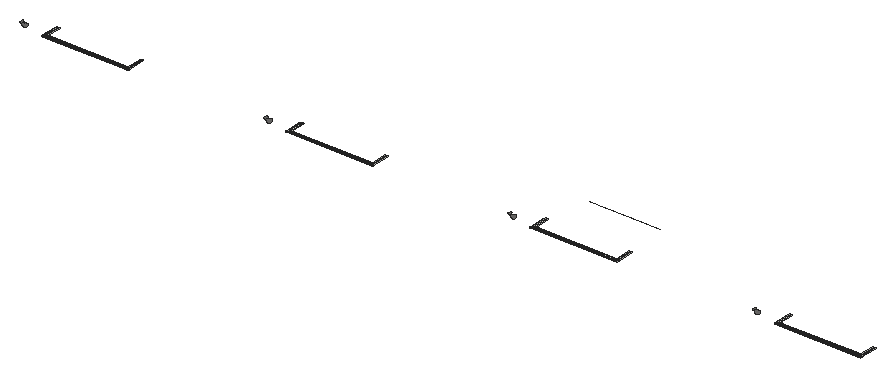
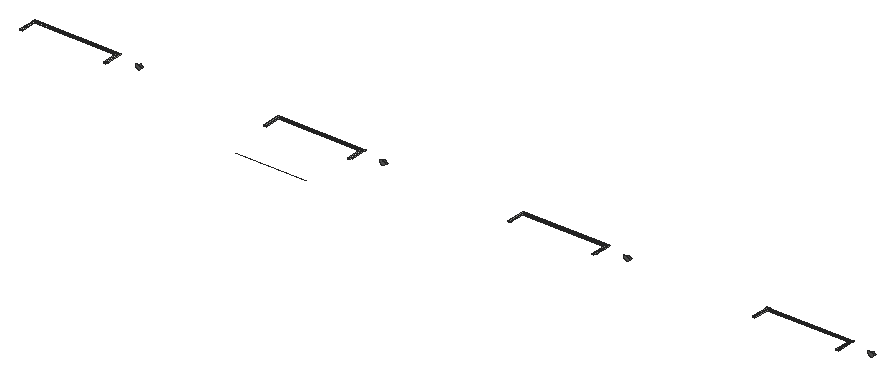
# SketchUp Ruby script. Lengths in inches.
U = 1.inch
M = Sketchup.active_model
def pt(a) = Geom::Point3d.new(a.map { |v| v * U })
def face(e, loops, mat)
  f = e.add_face(loops[0].map { |a| pt(a) })
  loops[1..].each { |l| e.add_face(l.map { |a| pt(a) }).erase! }
  f.material = f.back_material = mat if mat
  f
end
# faces: each face lists its corners as indices into pts; further lists are holes
def faces(e, pts, list, mat = nil) = list.each { |f| face(e, (f[0].is_a?(Array) ? f : [f]).map { |l| l.map { |i| pts[i] } }, mat) }
# xy, xz, yz: faces in a plane at the given z, y or x. An outline is a flat list of corners, or four numbers for a rectangle; further outlines are holes
def ring(l) = l.size == 4 ? [[l[0], l[1]], [l[2], l[1]], [l[2], l[3]], [l[0], l[3]]] : l.each_slice(2).to_a
def flat(e, list, mat, &to3) = list.each { |f| face(e, (f[0].is_a?(Array) ? f : [f]).map { |l| ring(l).map { |u, v| to3.(u, v) } }, mat) }
def xy(e, z, list, mat = nil) = flat(e, list, mat) { |x, y| [x, y, z] }
def xz(e, y, list, mat = nil) = flat(e, list, mat) { |x, z| [x, y, z] }
def yz(e, x, list, mat = nil) = flat(e, list, mat) { |y, z| [x, y, z] }
def lines(e, pts, list) = list.each { |a, b| e.add_line(pt(pts[a]), pt(pts[b])) }
# prism: a flat outline (further loops are holes) pulled along v
def prism(e, loops, v, mat = nil)
  f = face(e, loops, mat); d = Geom::Vector3d.new(v.map { |x| x * U })
  f.pushpull(f.normal.samedirection?(d) ? d.length : -d.length)
end
def box(e, o, s, mat = nil) = prism(e, [[o, [o[0] + s[0], o[1], o[2]], [o[0] + s[0], o[1] + s[1], o[2]], [o[0], o[1] + s[1], o[2]]]], [0, 0, s[2]], mat)
def at(x, y, z, deg = 0) = Geom::Transformation.translation(pt([x, y, z])) * Geom::Transformation.rotation(ORIGIN, Z_AXIS, deg.degrees)
def axes(o, x, y, z) = Geom::Transformation.new([*x, 0, *y, 0, *z, 0, *pt(o).to_a, 1])
def part(name) = M.definitions.add(name)
# library, detail: a bought-in or finely detailed component or shape, given as its bounding box
def library(name, o, s) = part(name).tap { |d| box(d.entities, o, s) }
def detail(e, o, s) = box(e.add_group.entities, o, s)
def put(e, d, t, mat = nil) = e.add_instance(d, t).tap { |i| i.material = mat if mat }
def group(e, t, mat = nil) = e.add_group.tap { |g| g.transformation = t; g.material = mat if mat }.entities
root = M.entities
M.materials.add("[0043_SaddleBrown]4").color = [124, 123, 122]
M.materials.add("[Granite Light Gray]").color = [149, 148, 144]
xy(root,289.5625,[[548.32,556.4375,551.76,559.875],[551.76,556.4375,990.19,559.875],[990.19,556.4375,992.12,559.875],[1798.95,556.4375,1802.38,559.875],[1802.38,556.4375,2240.81,559.875],
  [2240.81,556.4375,2242.75,559.875],[3049.57,556.4375,3053.01,559.875],[3053.01,556.4375,3491.44,559.875],[3491.44,556.4375,3493.37,559.875],[4300.2,556.4375,4303.63,559.875],
  [4303.63,556.4375,4742.06,559.875],[4742.06,556.4375,4744,559.875],[548.32,559.875,551.76,640.11],[551.76,559.875,551.76,651.03,563.08,651.03,563.08,571.2,978.86,571.2,978.86,651.03,990.19,651.03,990.19,559.875],[990.19,559.875,992.12,651.03],
  [1798.95,559.875,1802.38,640.11],[1802.38,559.875,1802.38,651.03,1813.71,651.03,1813.71,571.2,2229.49,571.2,2229.49,651.03,2240.81,651.03,2240.81,559.875],[2240.81,559.875,2242.75,651.03],[3049.57,559.875,3053.01,640.11],[3053.01,559.875,3053.01,651.03,3064.33,651.03,3064.33,571.2,3480.11,571.2,3480.11,651.03,3491.44,651.03,3491.44,559.875],
  [3491.44,559.875,3493.37,651.03],[4300.2,559.875,4303.63,640.11],[4303.63,559.875,4303.63,651.03,4314.96,651.03,4314.96,571.2,4730.74,571.2,4730.74,651.03,4742.06,651.03,4742.06,559.875],[4742.06,559.875,4744,651.03]])
xz(root,556.4375,[[548.32,289.5625,551.76,293],[990.19,289.5625,992.12,293],[1798.95,289.5625,1802.38,293],[2240.81,289.5625,2242.75,293],[3049.57,289.5625,3053.01,293],
  [3491.44,289.5625,3493.37,293],[4300.2,289.5625,4303.63,293],[4742.06,289.5625,4744,293]])
xz(root,556.4375,[[551.76,289.5625,990.19,293],[1802.38,289.5625,2240.81,293],[3053.01,289.5625,3491.44,293],[4303.63,289.5625,4742.06,293]],"[Granite Light Gray]")
xz(root,559.875,[[548.32,289.5625,551.76,293],[551.76,289.5625,990.19,293],[990.19,289.5625,992.12,293],[1798.95,289.5625,1802.38,293],[1802.38,289.5625,2240.81,293],
  [2240.81,289.5625,2242.75,293],[3049.57,289.5625,3053.01,293],[3053.01,289.5625,3491.44,293],[3491.44,289.5625,3493.37,293],[4300.2,289.5625,4303.63,293],
  [4303.63,289.5625,4742.06,293],[4742.06,289.5625,4744,293]])
xz(root,571.2,[[563.08,289.5625,978.86,293],[1813.71,289.5625,2229.49,293],[3064.33,289.5625,3480.11,293],[4314.96,289.5625,4730.74,293]])
xz(root,589.17,[[432.01,278.11,430.6,278.23,429.21,278.47,427.87,278.82,425.9375,279.59,424.24,280.61,422.86,281.85,421.82,283.26,421.19,284.78,420.98,286.37,421.19,287.95,421.82,289.48,422.86,290.88,424.24,292.125,425.9375,293.15,427.87,293.91,428.51,294.18,429.21,294.38,429.93,294.49,430.67,294.52,431.41,294.46,432.13,294.32,432.81,294.1,433.43,293.81,433.98,293.45,434.4375,293.03,434.8,292.56,435.06,292.06,435.42,291.61,435.7,291.13,435.875,290.63,435.95,290.11,435.93,289.59,435.8,289.08,435.58,288.59,435.26,288.125,434.85,287.7,434.37,287.32,433.8125,286.99,433.2,286.72,432.84,286.85,432.5,287,432.18,287.17,431.87,287.36,431.58,287.56,431.31,287.77,431.06,288,430.83,288.23,430.625,288.48,430.44,288.74,430.29,289.01,430.16,289.28,429.4,288.95,428.73,288.52,428.19,288.01,427.78,287.4375,427.54,286.82,427.45,286.18,427.54,285.53,427.78,284.92,428.19,284.34,428.73,283.83,429.4,283.4,430.16,283.07,431.09,283.04,432.03,283.07,432.95,283.14,433.87,283.27,434.77,283.44,435.66,283.67,436.51,283.93,437.34,284.25,438.13,284.61,438.88,285,439.59,285.44,440.25,285.92,440.84,286.83,441.3,287.79,441.65,288.76,441.875,289.76,441.97,290.77,441.94,291.78,441.79,292.78,441.51,293.77,441.11,294.74,440.59,295.68,439.96,296.58,439.21,297.43,439.98,297.24,440.76,297.1,441.55,297.01,442.36,296.97,443.16,296.98,443.97,297.04,444.76,297.14,445.54,297.3,446.29,297.51,447.02,297.76,447.71,298.06,448.37,298.4,448.37,289.47,448,288.82,447.62,288.18,447.23,287.54,446.8125,286.91,446.39,286.28,445.95,285.66,445.49,285.04,445.02,284.43,444.53,283.83,444.03,283.23,443.51,282.64,442.98,282.05,442.125,281.23,441.14,280.49,440.05,279.83,438.85,279.27,437.58,278.82,436.24,278.47,434.85,278.23,433.4375,278.11],[1682.64,278.11,1681.22,278.23,1679.84,278.47,1678.5,278.82,1676.5625,279.59,1674.87,280.61,1673.48,281.85,1672.45,283.26,1671.82,284.78,1671.6,286.37,1671.82,287.95,1672.45,289.48,1673.48,290.88,1674.87,292.125,1676.5625,293.15,1678.5,293.91,1679.14,294.18,1679.83,294.38,1680.56,294.49,1681.3,294.52,1682.04,294.46,1682.76,294.32,1683.43,294.1,1684.05,293.81,1684.6,293.45,1685.0625,293.03,1685.43,292.56,1685.68,292.06,1686.05,291.61,1686.32,291.13,1686.5,290.63,1686.58,290.11,1686.55,289.59,1686.43,289.08,1686.2,288.59,1685.88,288.125,1685.48,287.7,1684.99,287.32,1684.4375,286.99,1683.82,286.72,1683.47,286.85,1683.13,287,1682.8,287.17,1682.49,287.36,1682.2,287.56,1681.93,287.77,1681.68,288,1681.45,288.23,1681.25,288.48,1681.07,288.74,1680.91,289.01,1680.79,289.28,1680.02,288.95,1679.35,288.52,1678.81,288.01,1678.41,287.4375,1678.16,286.82,1678.08,286.18,1678.16,285.53,1678.41,284.92,1678.81,284.34,1679.35,283.83,1680.02,283.4,1680.79,283.07,1681.72,283.04,1682.65,283.07,1683.58,283.14,1684.5,283.27,1685.4,283.44,1686.28,283.67,1687.14,283.93,1687.96,284.25,1688.75,284.61,1689.51,285,1690.22,285.44,1690.88,285.92,1691.46,286.83,1691.93,287.79,1692.28,288.76,1692.5,289.76,1692.6,290.77,1692.57,291.78,1692.42,292.78,1692.14,293.77,1691.74,294.74,1691.22,295.68,1690.58,296.58,1689.84,297.43,1690.6,297.24,1691.38,297.1,1692.18,297.01,1692.98,296.97,1693.79,296.98,1694.59,297.04,1695.38,297.14,1696.16,297.3,1696.91,297.51,1697.64,297.76,1698.34,298.06,1698.99,298.4,1698.99,289.47,1698.625,288.82,1698.25,288.18,1697.85,287.54,1697.4375,286.91,1697.01,286.28,1696.57,285.66,1696.11,285.04,1695.64,284.43,1695.16,283.83,1694.65,283.23,1694.14,282.64,1693.61,282.05,1692.75,281.23,1691.77,280.49,1690.67,279.83,1689.48,279.27,1688.2,278.82,1686.86,278.47,1685.48,278.23,1684.0625,278.11],[2933.26,278.11,2931.85,278.23,2930.46,278.47,2929.12,278.82,2927.1875,279.59,2925.49,280.61,2924.11,281.85,2923.07,283.26,2922.44,284.78,2922.23,286.37,2922.44,287.95,2923.07,289.48,2924.11,290.88,2925.49,292.125,2927.1875,293.15,2929.12,293.91,2929.76,294.18,2930.46,294.38,2931.18,294.49,2931.92,294.52,2932.66,294.46,2933.38,294.32,2934.06,294.1,2934.68,293.81,2935.23,293.45,2935.6875,293.03,2936.05,292.56,2936.31,292.06,2936.67,291.61,2936.95,291.13,2937.125,290.63,2937.2,290.11,2937.18,289.59,2937.05,289.08,2936.83,288.59,2936.51,288.125,2936.1,287.7,2935.62,287.32,2935.0625,286.99,2934.45,286.72,2934.09,286.85,2933.75,287,2933.43,287.17,2933.12,287.36,2932.83,287.56,2932.56,287.77,2932.31,288,2932.08,288.23,2931.875,288.48,2931.69,288.74,2931.54,289.01,2931.41,289.28,2930.65,288.95,2929.98,288.52,2929.44,288.01,2929.03,287.4375,2928.79,286.82,2928.7,286.18,2928.79,285.53,2929.03,284.92,2929.44,284.34,2929.98,283.83,2930.65,283.4,2931.41,283.07,2932.34,283.04,2933.28,283.07,2934.2,283.14,2935.12,283.27,2936.02,283.44,2936.91,283.67,2937.76,283.93,2938.59,284.25,2939.38,284.61,2940.13,285,2940.84,285.44,2941.5,285.92,2942.09,286.83,2942.55,287.79,2942.9,288.76,2943.125,289.76,2943.22,290.77,2943.19,291.78,2943.04,292.78,2942.76,293.77,2942.36,294.74,2941.84,295.68,2941.21,296.58,2940.46,297.43,2941.23,297.24,2942.01,297.1,2942.8,297.01,2943.61,296.97,2944.41,296.98,2945.22,297.04,2946.01,297.14,2946.79,297.3,2947.54,297.51,2948.27,297.76,2948.96,298.06,2949.62,298.4,2949.62,289.47,2949.25,288.82,2948.87,288.18,2948.48,287.54,2948.0625,286.91,2947.64,286.28,2947.2,285.66,2946.74,285.04,2946.27,284.43,2945.78,283.83,2945.28,283.23,2944.76,282.64,2944.23,282.05,2943.375,281.23,2942.39,280.49,2941.3,279.83,2940.1,279.27,2938.83,278.82,2937.49,278.47,2936.1,278.23,2934.6875,278.11],[4183.89,278.11,4182.47,278.23,4181.09,278.47,4179.75,278.82,4177.8125,279.59,4176.12,280.61,4174.73,281.85,4173.7,283.26,4173.07,284.78,4172.85,286.37,4173.07,287.95,4173.7,289.48,4174.73,290.88,4176.12,292.125,4177.8125,293.15,4179.75,293.91,4180.39,294.18,4181.08,294.38,4181.81,294.49,4182.55,294.52,4183.29,294.46,4184.01,294.32,4184.68,294.1,4185.3,293.81,4185.85,293.45,4186.3125,293.03,4186.68,292.56,4186.93,292.06,4187.3,291.61,4187.57,291.13,4187.75,290.63,4187.83,290.11,4187.8,289.59,4187.68,289.08,4187.45,288.59,4187.13,288.125,4186.73,287.7,4186.24,287.32,4185.6875,286.99,4185.07,286.72,4184.72,286.85,4184.38,287,4184.05,287.17,4183.74,287.36,4183.45,287.56,4183.18,287.77,4182.93,288,4182.7,288.23,4182.5,288.48,4182.32,288.74,4182.16,289.01,4182.04,289.28,4181.27,288.95,4180.6,288.52,4180.06,288.01,4179.66,287.4375,4179.41,286.82,4179.33,286.18,4179.41,285.53,4179.66,284.92,4180.06,284.34,4180.6,283.83,4181.27,283.4,4182.04,283.07,4182.97,283.04,4183.9,283.07,4184.83,283.14,4185.75,283.27,4186.65,283.44,4187.53,283.67,4188.39,283.93,4189.21,284.25,4190,284.61,4190.76,285,4191.47,285.44,4192.13,285.92,4192.71,286.83,4193.18,287.79,4193.53,288.76,4193.75,289.76,4193.85,290.77,4193.82,291.78,4193.67,292.78,4193.39,293.77,4192.99,294.74,4192.47,295.68,4191.83,296.58,4191.09,297.43,4191.85,297.24,4192.63,297.1,4193.43,297.01,4194.23,296.97,4195.04,296.98,4195.84,297.04,4196.63,297.14,4197.41,297.3,4198.16,297.51,4198.89,297.76,4199.59,298.06,4200.24,298.4,4200.24,289.47,4199.875,288.82,4199.5,288.18,4199.1,287.54,4198.6875,286.91,4198.26,286.28,4197.82,285.66,4197.36,285.04,4196.89,284.43,4196.41,283.83,4195.9,283.23,4195.39,282.64,4194.86,282.05,4194,281.23,4193.02,280.49,4191.92,279.83,4190.73,279.27,4189.45,278.82,4188.11,278.47,4186.73,278.23,4185.3125,278.11],[416.49,289.66,415.94,290.04,415.39,290.41,414.82,290.77,414.24,291.13,413.66,291.48,413.0625,291.83,412.46,292.16,411.85,292.49,411.23,292.81,410.6,293.12,409.97,293.42,409.33,293.72,410.93,294.25,412.47,294.88,413.9375,295.59,415.32,296.39,416.62,297.25,417.8125,298.19,418.9,299.2,419.875,300.26,420.73,301.38,421.46,302.54,422.06,303.74,422.53,304.97,423.06,304.49,424.16,303.57,424.72,303.11,425.29,302.67,425.87,302.23,426.46,301.8,427.0625,301.37,427.67,300.95,428.29,300.54,428.92,300.13,429.5625,299.74,427.89,299.46,426.28,299.05,424.73,298.53,423.27,297.88,421.92,297.13,420.6875,296.27,419.59,295.33,418.64,294.3,417.84,293.21,417.22,292.0625,416.76,290.875],
  [1667.12,289.66,1666.57,290.04,1666.01,290.41,1664.87,291.13,1664.28,291.48,1663.6875,291.83,1663.09,292.16,1662.47,292.49,1661.86,292.81,1661.23,293.12,1660.6,293.42,1659.95,293.72,1661.56,294.25,1663.1,294.88,1664.5625,295.59,1665.95,296.39,1667.24,297.25,1668.4375,298.19,1669.52,299.2,1670.5,300.26,1671.36,301.38,1672.09,302.54,1672.69,303.74,1673.16,304.97,1673.69,304.49,1674.23,304.03,1674.78,303.57,1675.34,303.11,1675.91,302.67,1676.5,302.23,1677.09,301.8,1677.6875,301.37,1678.3,300.95,1678.92,300.54,1679.55,300.13,1680.1875,299.74,1678.52,299.46,1676.9,299.05,1675.36,298.53,1673.9,297.88,1672.55,297.13,1671.3125,296.27,1670.21,295.33,1669.26,294.3,1668.47,293.21,1667.84,292.0625,1667.39,290.875],[2917.74,289.66,2917.19,290.04,2916.64,290.41,2916.07,290.77,2915.49,291.13,2914.91,291.48,2914.3125,291.83,2913.71,292.16,2913.1,292.49,2912.48,292.81,2911.85,293.12,2911.22,293.42,2910.58,293.72,2912.18,294.25,2913.72,294.88,2915.1875,295.59,2916.57,296.39,2917.87,297.25,2919.0625,298.19,2920.15,299.2,2921.125,300.26,2921.98,301.38,2922.71,302.54,2923.31,303.74,2923.78,304.97,2924.31,304.49,2925.41,303.57,2925.97,303.11,2926.54,302.67,2927.12,302.23,2927.71,301.8,2928.3125,301.37,2928.92,300.95,2929.54,300.54,2930.17,300.13,2930.8125,299.74,2929.14,299.46,2927.53,299.05,2925.98,298.53,2924.52,297.88,2923.17,297.13,2921.9375,296.27,2920.84,295.33,2919.89,294.3,2919.09,293.21,2918.47,292.0625,2918.01,290.875],[4168.37,289.66,4167.82,290.04,4167.26,290.41,4166.12,291.13,4165.53,291.48,4164.9375,291.83,4164.34,292.16,4163.72,292.49,4163.11,292.81,4162.48,293.12,4161.85,293.42,4161.2,293.72,4162.81,294.25,4164.35,294.88,4165.8125,295.59,4167.2,296.39,4168.49,297.25,4169.6875,298.19,4170.77,299.2,4171.75,300.26,4172.61,301.38,4173.34,302.54,4173.94,303.74,4174.41,304.97,4174.94,304.49,4175.48,304.03,4176.03,303.57,4176.59,303.11,4177.16,302.67,4177.75,302.23,4178.34,301.8,4178.9375,301.37,4179.55,300.95,4180.17,300.54,4180.8,300.13,4181.4375,299.74,4179.77,299.46,4178.15,299.05,4176.61,298.53,4175.15,297.88,4173.8,297.13,4172.5625,296.27,4171.46,295.33,4170.51,294.3,4169.72,293.21,4169.09,292.0625,4168.64,290.875]],"[0043_SaddleBrown]4")
xz(root,640.11,[[548.32,289.5625,551.76,293],[1798.95,289.5625,1802.38,293],[3049.57,289.5625,3053.01,293],[4300.2,289.5625,4303.63,293]])
xz(root,651.03,[[551.76,289.5625,563.08,293],[978.86,289.5625,990.19,293],[990.19,289.5625,992.12,293],[1802.38,289.5625,1813.71,293],[2229.49,289.5625,2240.81,293],
  [2240.81,289.5625,2242.75,293],[3053.01,289.5625,3064.33,293],[3480.11,289.5625,3491.44,293],[3491.44,289.5625,3493.37,293],[4303.63,289.5625,4314.96,293],
  [4730.74,289.5625,4742.06,293],[4742.06,289.5625,4744,293]])
yz(root,548.32,[[556.4375,289.5625,559.875,293],[559.875,289.5625,640.11,293]])
yz(root,551.76,[[556.4375,289.5625,559.875,293],[559.875,289.5625,640.11,293],[640.11,289.5625,651.03,293]])
yz(root,563.08,[[571.2,289.5625,651.03,293]])
yz(root,978.86,[[571.2,289.5625,651.03,293]])
yz(root,990.19,[[556.4375,289.5625,559.875,293],[559.875,289.5625,651.03,293]])
yz(root,992.12,[[556.4375,289.5625,559.875,293],[559.875,289.5625,651.03,293]])
yz(root,1798.95,[[556.4375,289.5625,559.875,293],[559.875,289.5625,640.11,293]])
yz(root,1802.38,[[556.4375,289.5625,559.875,293],[559.875,289.5625,640.11,293],[640.11,289.5625,651.03,293]])
yz(root,1813.71,[[571.2,289.5625,651.03,293]])
yz(root,2229.49,[[571.2,289.5625,651.03,293]])
yz(root,2240.81,[[556.4375,289.5625,559.875,293],[559.875,289.5625,651.03,293]])
yz(root,2242.75,[[556.4375,289.5625,559.875,293],[559.875,289.5625,651.03,293]])
yz(root,3049.57,[[556.4375,289.5625,559.875,293],[559.875,289.5625,640.11,293]])
yz(root,3053.01,[[556.4375,289.5625,559.875,293],[559.875,289.5625,640.11,293],[640.11,289.5625,651.03,293]])
yz(root,3064.33,[[571.2,289.5625,651.03,293]])
yz(root,3480.11,[[571.2,289.5625,651.03,293]])
yz(root,3491.44,[[556.4375,289.5625,559.875,293],[559.875,289.5625,651.03,293]])
yz(root,3493.37,[[556.4375,289.5625,559.875,293],[559.875,289.5625,651.03,293]])
yz(root,4300.2,[[556.4375,289.5625,559.875,293],[559.875,289.5625,640.11,293]])
yz(root,4303.63,[[556.4375,289.5625,559.875,293],[559.875,289.5625,640.11,293],[640.11,289.5625,651.03,293]])
yz(root,4314.96,[[571.2,289.5625,651.03,293]])
yz(root,4730.74,[[571.2,289.5625,651.03,293]])
yz(root,4742.06,[[556.4375,289.5625,559.875,293],[559.875,289.5625,651.03,293]])
yz(root,4744,[[556.4375,289.5625,559.875,293],[559.875,289.5625,651.03,293]])
p = [[3452.21,884.37,280.38],[3089.42,884.37,280.38]]
lines(root,p,[[0,1]])
